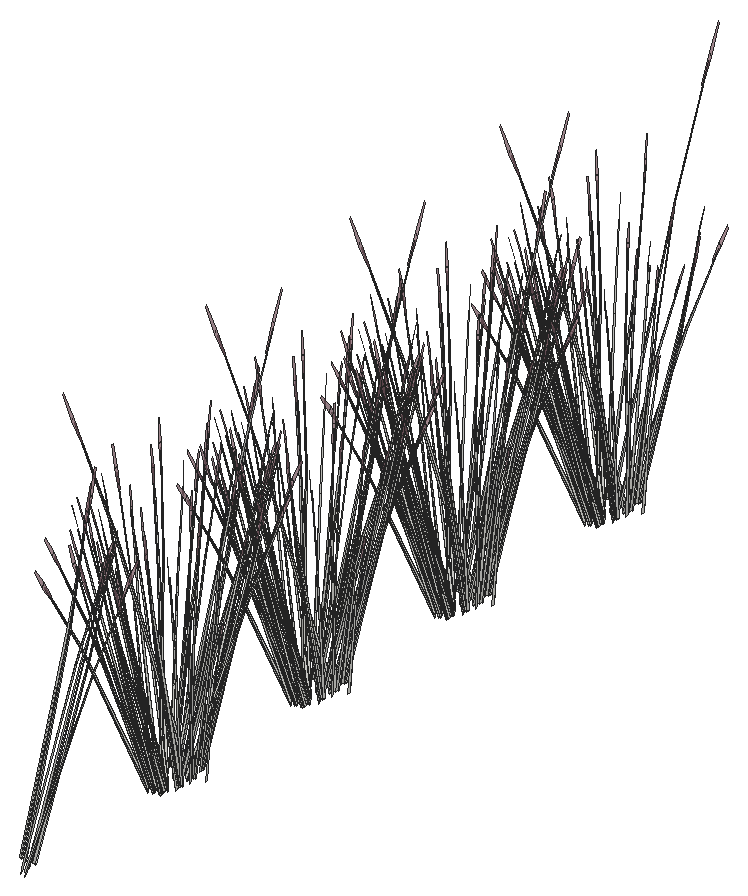
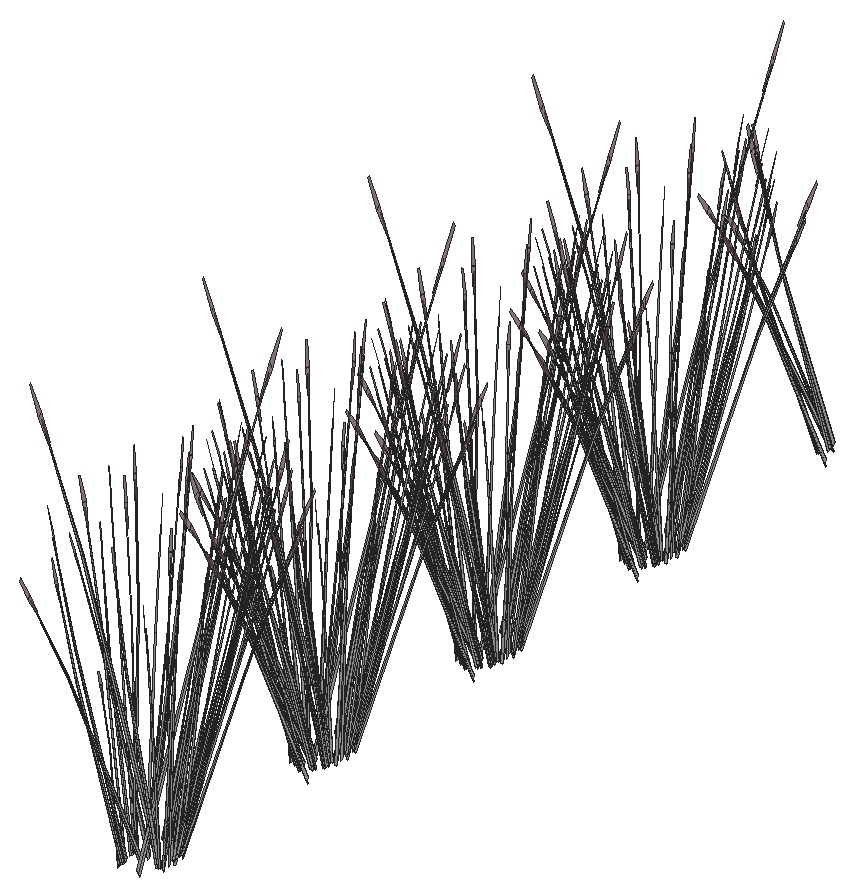
# SketchUp Ruby script. Lengths in inches.
U = 1.inch
M = Sketchup.active_model
def pt(a) = Geom::Point3d.new(a.map { |v| v * U })
def face(e, loops, mat)
  f = e.add_face(loops[0].map { |a| pt(a) })
  loops[1..].each { |l| e.add_face(l.map { |a| pt(a) }).erase! }
  f.material = f.back_material = mat if mat
  f
end
# faces: each face lists its corners as indices into pts; further lists are holes
def faces(e, pts, list, mat = nil) = list.each { |f| face(e, (f[0].is_a?(Array) ? f : [f]).map { |l| l.map { |i| pts[i] } }, mat) }
# xy, xz, yz: faces in a plane at the given z, y or x. An outline is a flat list of corners, or four numbers for a rectangle; further outlines are holes
def ring(l) = l.size == 4 ? [[l[0], l[1]], [l[2], l[1]], [l[2], l[3]], [l[0], l[3]]] : l.each_slice(2).to_a
def flat(e, list, mat, &to3) = list.each { |f| face(e, (f[0].is_a?(Array) ? f : [f]).map { |l| ring(l).map { |u, v| to3.(u, v) } }, mat) }
def xy(e, z, list, mat = nil) = flat(e, list, mat) { |x, y| [x, y, z] }
def xz(e, y, list, mat = nil) = flat(e, list, mat) { |x, z| [x, y, z] }
def yz(e, x, list, mat = nil) = flat(e, list, mat) { |y, z| [x, y, z] }
def lines(e, pts, list) = list.each { |a, b| e.add_line(pt(pts[a]), pt(pts[b])) }
# prism: a flat outline (further loops are holes) pulled along v
def prism(e, loops, v, mat = nil)
  f = face(e, loops, mat); d = Geom::Vector3d.new(v.map { |x| x * U })
  f.pushpull(f.normal.samedirection?(d) ? d.length : -d.length)
end
def box(e, o, s, mat = nil) = prism(e, [[o, [o[0] + s[0], o[1], o[2]], [o[0] + s[0], o[1] + s[1], o[2]], [o[0], o[1] + s[1], o[2]]]], [0, 0, s[2]], mat)
def at(x, y, z, deg = 0) = Geom::Transformation.translation(pt([x, y, z])) * Geom::Transformation.rotation(ORIGIN, Z_AXIS, deg.degrees)
def axes(o, x, y, z) = Geom::Transformation.new([*x, 0, *y, 0, *z, 0, *pt(o).to_a, 1])
def part(name) = M.definitions.add(name)
# library, detail: a bought-in or finely detailed component or shape, given as its bounding box
def library(name, o, s) = part(name).tap { |d| box(d.entities, o, s) }
def detail(e, o, s) = box(e.add_group.entities, o, s)
def put(e, d, t, mat = nil) = e.add_instance(d, t).tap { |i| i.material = mat if mat }
def group(e, t, mat = nil) = e.add_group.tap { |g| g.transformation = t; g.material = mat if mat }.entities
root = M.entities
M.materials.add("LightPink_Translucent").color = [144, 107, 117]
M.materials["LightPink_Translucent"].alpha = 0.75
c1 = part("blade")
p = [[2.15,0.21,22],[0,0.17,0],[0.09,0.45,0],[2.18,0.31,22],[2.29,0.31,22],[0.38,0.45,0],
  [2.48,0.24,33],[2.49,0.24,33],[2.48,0.22,33]]
faces(c1.entities,p,[[0,1,2,3],[4,5,2,3],[6,3,4,7],[8,0,3,6]])
c2 = part("seeds")
p = [[0.3,-0.1,1.38],[-0.01,-0.03,1.59],[-0.01,-0.03,0.03],[0.14,-0.07,-0.07],[0.29,-0.03,3],[0.15,0.01,3.11]]
faces(c2.entities,p,[[0,1,2,3],[1,0,4,5]],"LightPink_Translucent")
c3 = part("blade with seeds")
put(c3.entities,c1,at(0,0,0))
put(c3.entities,c2,axes([2.4,0.25,30.99],[1.5799,-0.05474,1.17369],[-0.12525,1.92788,0.29478],[-0.07173,-0.02425,1.56792]))
put(root,c3,axes([251.06,64.61,2.83],[0.18323,0.41084,-0.41166],[-0.19356,0.3598,-0.31887],[-0.02788,0.20874,0.78768]))
put(root,c3,axes([251.6,65,2.59],[0.25161,0.15328,-0.37087],[-0.08624,0.52553,-0.28727],[0.02307,0.21159,0.70962]))
put(root,c3,axes([251.74,63.92,2.01],[-0.05851,-0.19632,1.24382],[0.27036,-0.16528,0.10057],[0.0611,0.3082,0.53172]))
put(root,c3,axes([251.48,65.33,2.48],[-0.07716,0.47021,-0.25703],[-0.22512,-0.13715,0.33183],[0.02064,0.18932,0.63492]))
put(root,c3,axes([251,64.42,3.07],[-0.00666,0.56559,-0.57235],[-0.28045,-0.03799,0.06907],[-0.0296,0.23961,0.80965]))
put(root,c3,axes([251.26,64.02,2.01],[-0.00626,-0.23468,1.24382],[0.27152,0.15569,0.10057],[-0.01679,0.33444,0.53172]))
put(root,c3,axes([250.9,65.21,1.63],[0.00562,-0.31565,1.12021],[0.25293,0.16673,0.1548],[-0.02192,0.33641,0.52896]))
put(root,c3,axes([251.1,79.1,2.01],[0.05851,0.19632,1.24382],[-0.27036,0.16528,0.10057],[-0.0611,-0.3082,0.53172]))
put(root,c3,axes([251.84,78.82,2.48],[0.07716,-0.47021,-0.25703],[0.22512,0.13715,0.33183],[-0.02064,-0.18932,0.63492]))
put(root,c3,axes([252.01,79.45,2.01],[-0.04766,0.21017,1.24382],[-0.19993,-0.43493,0.10057],[0.09019,-0.27107,0.53172]))
put(root,c3,axes([251.73,79.15,2.59],[-0.25161,-0.15328,-0.37087],[0.08624,-0.52553,-0.28727],[-0.02307,-0.21159,0.70962]))
put(root,c3,axes([252.27,79.54,2.59],[-0.18323,-0.41084,-0.37087],[0.19356,-0.3598,-0.28727],[0.02788,-0.20874,0.70962]))
put(root,c3,axes([251.94,79.12,2.85],[-0.25047,0.28468,-0.08826],[-0.12309,-0.50526,-0.48986],[-0.03305,-0.21292,0.74434]))
put(root,c3,axes([252.46,79.76,2.85],[-0.2813,-0.0303,-0.08826],[0.00769,-0.57361,-0.48986],[0.01954,-0.22092,0.74434]))
put(root,c3,axes([252.44,79.39,2.48],[0.17318,-0.32193,-0.25703],[0.16394,0.36759,0.33183],[0.02494,-0.18677,0.63492]))
put(root,c3,axes([251.19,79,2.48],[-0.03953,-0.49251,-0.25703],[0.22598,-0.13005,0.33183],[-0.0607,-0.14114,0.63492]))
put(root,c3,axes([250.71,79.71,2.01],[0.09507,0.10535,1.24382],[-0.19675,0.44195,0.10057],[-0.12263,-0.19937,0.53172]))
put(root,c3,axes([251.17,79.4,2.59],[-0.25257,0.14535,-0.37087],[-0.04418,-0.55045,-0.28727],[-0.06784,-0.15774,0.70962]))
put(root,c3,axes([252.65,80.49,2.59],[-0.06575,-0.55831,-0.37087],[0.24901,-0.09767,-0.28727],[0.07136,-0.14996,0.70962]))
put(root,c3,axes([252.77,80.89,2.85],[-0.23676,-0.33715,-0.08826],[0.1364,-0.48826,-0.48986],[0.06689,-0.16972,0.74434]))
put(root,c3,axes([251.79,82.73,1.61],[0.22119,0.24656,1.09782],[-0.21669,0.53118,0.43413],[-0.09706,-0.31482,0.92034]))
put(root,c3,axes([252.84,80.55,2.48],[0.2228,-0.08739,-0.25703],[0.05883,0.49954,0.33183],[0.06385,-0.13418,0.63492]))
put(root,c3,axes([250.67,79.86,2.48],[-0.14563,-0.38283,-0.25703],[0.16629,-0.3624,0.33183],[-0.08449,-0.05514,0.63492]))
put(root,c3,axes([250.74,80.24,2.59],[-0.18586,0.40503,-0.37087],[-0.16277,-0.42787,-0.28727],[-0.09443,-0.06163,0.70962]))
put(root,c3,axes([250.84,79.82,2.85],[-0.0137,0.62183,-0.08826],[-0.25949,-0.017,-0.48986],[-0.09994,-0.0432,0.74434]))
put(root,c3,axes([252.78,82.21,2.85],[-0.12878,-0.55367,-0.08826],[0.22857,-0.27208,-0.48986],[0.09632,-0.07305,0.74434]))
put(root,c3,axes([252.77,81.73,2.59],[0.06934,-0.55619,-0.37087],[0.23774,0.19064,-0.28727],[0.09572,-0.051,0.70962]))
put(root,c3,axes([250.51,80.68,2.01],[0.10617,-0.01385,1.24382],[-0.07043,0.60021,0.10057],[-0.1513,-0.03712,0.53172]))
put(root,c3,axes([252.91,81.98,2.48],[0.21272,0.17057,-0.25703],[-0.06204,0.49764,0.33183],[0.08564,-0.04563,0.63492]))
put(root,c3,axes([250.41,81.19,2.48],[-0.21272,-0.17057,-0.25703],[0.06204,-0.49764,0.33183],[-0.08564,0.04563,0.63492]))
put(root,c3,axes([252.33,81.37,2.01],[-0.10617,0.01385,1.24382],[0.07043,-0.60021,0.10057],[0.1513,0.03712,0.53172]))
put(root,c3,axes([251.0625,81.11,1.62],[0.07276,-0.08845,1.2851],[0.02509,0.61759,0.10057],[-0.15759,0.08195,0.4593]))
put(root,c3,axes([250.56,81.44,2.59],[-0.06934,0.55619,-0.37087],[-0.23774,-0.19064,-0.28727],[-0.09572,0.051,0.70962]))
put(root,c3,axes([250.55,80.97,2.85],[0.12878,0.55367,-0.08826],[-0.22857,0.27208,-0.48986],[-0.09632,0.07305,0.74434]))
put(root,c3,axes([253.09,83.37,2.04],[-0.04899,-0.514,-0.02534],[0.23154,-0.11817,-0.1149],[0.04835,0.03259,0.37899]))
put(root,c3,axes([252.49,83.36,2.85],[0.0137,-0.62183,-0.08826],[0.25949,0.017,-0.48986],[0.09994,0.0432,0.74434]))
put(root,c3,axes([250.55,81.73,2.01],[0.08881,-0.12933,1.24382],[0.07477,0.59764,0.10057],[-0.13942,0.13507,0.53172]))
put(root,c3,axes([252.66,83.3125,2.48],[0.14563,0.38283,-0.25703],[-0.16629,0.3624,0.33183],[0.08449,0.05514,0.63492]))
put(root,c3,axes([250.49,82.625,2.48],[-0.2228,0.08739,-0.25703],[-0.05883,-0.49954,0.33183],[-0.06385,0.13418,0.63492]))
put(root,c3,axes([252.13,82.33,2.01],[-0.09507,-0.10535,1.24382],[0.19675,-0.44195,0.10057],[0.12263,0.19937,0.53172]))
put(root,c3,axes([252.15,80.94,2.44],[-0.22117,-0.3177,1.00363],[0.23354,-0.49464,0.43304],[0.07136,0.29809,0.97011]))
put(root,c3,axes([250.56,82.28,2.85],[0.23676,0.33715,-0.08826],[-0.1364,0.48826,-0.48986],[-0.06689,0.16972,0.74434]))
put(root,c3,axes([251.98,84.03,2.85],[0.15252,-0.52338,-0.08826],[0.22088,0.30152,-0.48986],[0.07678,0.14787,0.74434]))
put(root,c3,axes([250.875,82.13,2.01],[0.06393,-0.18788,1.24382],[0.16142,0.50711,0.10057],[-0.11071,0.23094,0.53172]))
put(root,c3,axes([250.67,82.68,2.59],[0.06575,0.55831,-0.37087],[-0.24901,0.09767,-0.28727],[-0.07136,0.14996,0.70962]))
put(root,c3,axes([252.16,83.77,2.59],[0.25257,-0.14535,-0.37087],[0.04418,0.55045,-0.28727],[0.06784,0.15774,0.70962]))
put(root,c3,axes([250.83,82.6,2.01],[0.04766,-0.21017,1.24382],[0.19993,0.43493,0.10057],[-0.09019,0.27107,0.53172]))
put(root,c3,axes([250.88,83.78,2.48],[-0.17318,0.32193,-0.25703],[-0.16394,-0.36759,0.33183],[-0.02494,0.18677,0.63492]))
put(root,c3,axes([251.38,84.05,2.85],[0.25047,-0.28468,-0.08826],[0.12309,0.50526,-0.48986],[0.03305,0.21292,0.74434]))
put(root,c3,axes([251.06,83.63,2.83],[0.18323,0.41084,-0.41166],[-0.19356,0.3598,-0.31887],[-0.02788,0.20874,0.78768]))
put(root,c3,axes([251.6,84.03,2.59],[0.25161,0.15328,-0.37087],[-0.08624,0.52553,-0.28727],[0.02307,0.21159,0.70962]))
put(root,c3,axes([251.74,82.94,2.01],[-0.05851,-0.19632,1.24382],[0.27036,-0.16528,0.10057],[0.0611,0.3082,0.53172]))
put(root,c3,axes([251.48,84.35,2.48],[-0.07716,0.47021,-0.25703],[-0.22512,-0.13715,0.33183],[0.02064,0.18932,0.63492]))
put(root,c3,axes([251,83.44,3.07],[-0.00666,0.56559,-0.57235],[-0.28045,-0.03799,0.06907],[-0.0296,0.23961,0.80965]))
put(root,c3,axes([251.26,83.04,2.01],[-0.00626,-0.23468,1.24382],[0.27152,0.15569,0.10057],[-0.01679,0.33444,0.53172]))
put(root,c3,axes([250.9,84.24,1.63],[0.00562,-0.31565,1.12021],[0.25293,0.16673,0.1548],[-0.02192,0.33641,0.52896]))
put(root,c3,axes([251.1,95.68,2.01],[0.05851,0.19632,1.24382],[-0.27036,0.16528,0.10057],[-0.0611,-0.3082,0.53172]))
put(root,c3,axes([251.82,95.82,2.81],[-0.12216,-0.49718,-0.51563],[0.25147,-0.27708,0.06223],[-0.02857,-0.24022,0.72942]))
put(root,c3,axes([252.33,96.31,2.81],[0.00666,-0.56559,-0.51563],[0.28045,0.03799,0.06223],[0.0296,-0.23961,0.72942]))
put(root,c3,axes([251.84,95.4,2.48],[0.07716,-0.47021,-0.25703],[0.22512,0.13715,0.33183],[-0.02064,-0.18932,0.63492]))
put(root,c3,axes([252.01,96.02,2.01],[-0.04766,0.21017,1.24382],[-0.19993,-0.43493,0.10057],[0.09019,-0.27107,0.53172]))
put(root,c3,axes([251.73,95.72,2.59],[-0.25161,-0.15328,-0.37087],[0.08624,-0.52553,-0.28727],[-0.02307,-0.21159,0.70962]))
put(root,c3,axes([252.27,96.12,2.59],[-0.18323,-0.41084,-0.37087],[0.19356,-0.3598,-0.28727],[0.02788,-0.20874,0.70962]))
put(root,c3,axes([251.94,95.7,2.85],[-0.25047,0.28468,-0.08826],[-0.12309,-0.50526,-0.48986],[-0.03305,-0.21292,0.74434]))
put(root,c3,axes([252.46,96.34,2.85],[-0.2813,-0.0303,-0.08826],[0.00769,-0.57361,-0.48986],[0.01954,-0.22092,0.74434]))
put(root,c3,axes([252.44,95.97,2.48],[0.17318,-0.32193,-0.25703],[0.16394,0.36759,0.33183],[0.02494,-0.18677,0.63492]))
put(root,c3,axes([251.19,95.57,2.48],[-0.03953,-0.49251,-0.25703],[0.22598,-0.13005,0.33183],[-0.0607,-0.14114,0.63492]))
put(root,c3,axes([250.71,96.29,2.01],[0.09507,0.10535,1.24382],[-0.19675,0.44195,0.10057],[-0.12263,-0.19937,0.53172]))
put(root,c3,axes([251.17,95.98,2.59],[-0.25257,0.14535,-0.37087],[-0.04418,-0.55045,-0.28727],[-0.06784,-0.15774,0.70962]))
put(root,c3,axes([252.65,97.07,2.59],[-0.06575,-0.55831,-0.37087],[0.24901,-0.09767,-0.28727],[0.07136,-0.14996,0.70962]))
put(root,c3,axes([252.77,97.47,2.85],[-0.23676,-0.33715,-0.08826],[0.1364,-0.48826,-0.48986],[0.06689,-0.16972,0.74434]))
put(root,c3,axes([251.79,99.31,1.61],[0.22119,0.24656,1.09782],[-0.21669,0.53118,0.43413],[-0.09706,-0.31482,0.92034]))
put(root,c3,axes([252.84,97.125,2.48],[0.2228,-0.08739,-0.25703],[0.05883,0.49954,0.33183],[0.06385,-0.13418,0.63492]))
put(root,c3,axes([250.67,96.4375,2.48],[-0.14563,-0.38283,-0.25703],[0.16629,-0.3624,0.33183],[-0.08449,-0.05514,0.63492]))
put(root,c3,axes([250.74,96.82,2.59],[-0.18586,0.40503,-0.37087],[-0.16277,-0.42787,-0.28727],[-0.09443,-0.06163,0.70962]))
put(root,c3,axes([250.84,96.4,2.85],[-0.0137,0.62183,-0.08826],[-0.25949,-0.017,-0.48986],[-0.09994,-0.0432,0.74434]))
put(root,c3,axes([252.78,98.78,2.85],[-0.12878,-0.55367,-0.08826],[0.22857,-0.27208,-0.48986],[0.09632,-0.07305,0.74434]))
put(root,c3,axes([252.77,98.31,2.59],[0.06934,-0.55619,-0.37087],[0.23774,0.19064,-0.28727],[0.09572,-0.051,0.70962]))
put(root,c3,axes([250.51,97.25,2.01],[0.10617,-0.01385,1.24382],[-0.07043,0.60021,0.10057],[-0.1513,-0.03712,0.53172]))
put(root,c3,axes([252.91,98.5625,2.48],[0.21272,0.17057,-0.25703],[-0.06204,0.49764,0.33183],[0.08564,-0.04563,0.63492]))
put(root,c3,axes([250.41,97.77,2.48],[-0.21272,-0.17057,-0.25703],[0.06204,-0.49764,0.33183],[-0.08564,0.04563,0.63492]))
put(root,c3,axes([252.33,97.94,2.01],[-0.10617,0.01385,1.24382],[0.07043,-0.60021,0.10057],[0.1513,0.03712,0.53172]))
put(root,c3,axes([251.0625,97.69,1.62],[0.07276,-0.08845,1.2851],[0.02509,0.61759,0.10057],[-0.15759,0.08195,0.4593]))
put(root,c3,axes([250.56,98.02,2.59],[-0.06934,0.55619,-0.37087],[-0.23774,-0.19064,-0.28727],[-0.09572,0.051,0.70962]))
put(root,c3,axes([250.55,97.55,2.85],[0.12878,0.55367,-0.08826],[-0.22857,0.27208,-0.48986],[-0.09632,0.07305,0.74434]))
put(root,c3,axes([253.09,99.95,2.04],[-0.04899,-0.514,-0.02534],[0.23154,-0.11817,-0.1149],[0.04835,0.03259,0.37899]))
put(root,c3,axes([252.49,99.93,2.85],[0.0137,-0.62183,-0.08826],[0.25949,0.017,-0.48986],[0.09994,0.0432,0.74434]))
put(root,c3,axes([250.55,98.31,2.01],[0.08881,-0.12933,1.24382],[0.07477,0.59764,0.10057],[-0.13942,0.13507,0.53172]))
put(root,c3,axes([252.5,99.63,2.81],[0.25586,0.01472,-0.51563],[-0.01718,0.61995,0.06223],[0.1084,0.06542,0.72942]))
put(root,c3,axes([252.66,99.89,2.48],[0.14563,0.38283,-0.25703],[-0.16629,0.3624,0.33183],[0.08449,0.05514,0.63492]))
put(root,c3,axes([250.49,99.2,2.48],[-0.2228,0.08739,-0.25703],[-0.05883,-0.49954,0.33183],[-0.06385,0.13418,0.63492]))
put(root,c3,axes([252.13,98.91,2.01],[-0.09507,-0.10535,1.24382],[0.19675,-0.44195,0.10057],[0.12263,0.19937,0.53172]))
put(root,c3,axes([252.15,97.52,2.44],[-0.22117,-0.3177,1.00363],[0.23354,-0.49464,0.43304],[0.07136,0.29809,0.97011]))
put(root,c3,axes([250.56,98.86,2.85],[0.23676,0.33715,-0.08826],[-0.1364,0.48826,-0.48986],[-0.06689,0.16972,0.74434]))
put(root,c3,axes([251.98,100.61,2.85],[0.15252,-0.52338,-0.08826],[0.22088,0.30152,-0.48986],[0.07678,0.14787,0.74434]))
put(root,c3,axes([250.875,98.71,2.01],[0.06393,-0.18788,1.24382],[0.16142,0.50711,0.10057],[-0.11071,0.23094,0.53172]))
put(root,c3,axes([250.67,99.26,2.59],[0.06575,0.55831,-0.37087],[-0.24901,0.09767,-0.28727],[-0.07136,0.14996,0.70962]))
put(root,c3,axes([252.16,100.35,2.59],[0.25257,-0.14535,-0.37087],[0.04418,0.55045,-0.28727],[0.06784,0.15774,0.70962]))
put(root,c3,axes([250.83,99.17,2.01],[0.04766,-0.21017,1.24382],[0.19993,0.43493,0.10057],[-0.09019,0.27107,0.53172]))
put(root,c3,axes([250.88,100.36,2.48],[-0.17318,0.32193,-0.25703],[-0.16394,-0.36759,0.33183],[-0.02494,0.18677,0.63492]))
put(root,c3,axes([251.38,100.63,2.85],[0.25047,-0.28468,-0.08826],[0.12309,0.50526,-0.48986],[0.03305,0.21292,0.74434]))
put(root,c3,axes([251.06,100.21,2.83],[0.18323,0.41084,-0.41166],[-0.19356,0.3598,-0.31887],[-0.02788,0.20874,0.78768]))
put(root,c3,axes([251.6,100.61,2.59],[0.25161,0.15328,-0.37087],[-0.08624,0.52553,-0.28727],[0.02307,0.21159,0.70962]))
put(root,c3,axes([251.74,99.52,2.01],[-0.05851,-0.19632,1.24382],[0.27036,-0.16528,0.10057],[0.0611,0.3082,0.53172]))
put(root,c3,axes([251.48,100.93,2.48],[-0.07716,0.47021,-0.25703],[-0.22512,-0.13715,0.33183],[0.02064,0.18932,0.63492]))
put(root,c3,axes([251,100.02,3.07],[-0.00666,0.56559,-0.57235],[-0.28045,-0.03799,0.06907],[-0.0296,0.23961,0.80965]))
put(root,c3,axes([251.26,99.62,2.01],[-0.00626,-0.23468,1.24382],[0.27152,0.15569,0.10057],[-0.01679,0.33444,0.53172]))
put(root,c3,axes([250.9,100.82,1.63],[0.00562,-0.31565,1.12021],[0.25293,0.16673,0.1548],[-0.02192,0.33641,0.52896]))
put(root,c3,axes([251.1,112.43,2.01],[0.05851,0.19632,1.24382],[-0.27036,0.16528,0.10057],[-0.0611,-0.3082,0.53172]))
put(root,c3,axes([251.82,112.58,2.81],[-0.12216,-0.49718,-0.51563],[0.25147,-0.27708,0.06223],[-0.02857,-0.24022,0.72942]))
put(root,c3,axes([252.33,113.06,2.81],[0.00666,-0.56559,-0.51563],[0.28045,0.03799,0.06223],[0.0296,-0.23961,0.72942]))
put(root,c3,axes([251.84,112.16,2.48],[0.07716,-0.47021,-0.25703],[0.22512,0.13715,0.33183],[-0.02064,-0.18932,0.63492]))
put(root,c3,axes([252.01,112.78,2.01],[-0.04766,0.21017,1.24382],[-0.19993,-0.43493,0.10057],[0.09019,-0.27107,0.53172]))
put(root,c3,axes([251.73,112.48,2.59],[-0.25161,-0.15328,-0.37087],[0.08624,-0.52553,-0.28727],[-0.02307,-0.21159,0.70962]))
put(root,c3,axes([252.27,112.875,2.59],[-0.18323,-0.41084,-0.37087],[0.19356,-0.3598,-0.28727],[0.02788,-0.20874,0.70962]))
put(root,c3,axes([251.94,112.45,2.85],[-0.25047,0.28468,-0.08826],[-0.12309,-0.50526,-0.48986],[-0.03305,-0.21292,0.74434]))
put(root,c3,axes([252.46,113.09,2.85],[-0.2813,-0.0303,-0.08826],[0.00769,-0.57361,-0.48986],[0.01954,-0.22092,0.74434]))
put(root,c3,axes([252.44,112.72,2.48],[0.17318,-0.32193,-0.25703],[0.16394,0.36759,0.33183],[0.02494,-0.18677,0.63492]))
put(root,c3,axes([251.27,112.72,2.81],[-0.21825,-0.29555,-0.51563],[0.15511,-0.5179,0.06223],[-0.07907,-0.17646,0.72942]))
put(root,c3,axes([251.19,112.33,2.48],[-0.03953,-0.49251,-0.25703],[0.22598,-0.13005,0.33183],[-0.0607,-0.14114,0.63492]))
put(root,c3,axes([250.71,113.04,2.01],[0.09507,0.10535,1.24382],[-0.19675,0.44195,0.10057],[-0.12263,-0.19937,0.53172]))
put(root,c3,axes([251.17,112.73,2.59],[-0.25257,0.14535,-0.37087],[-0.04418,-0.55045,-0.28727],[-0.06784,-0.15774,0.70962]))
put(root,c3,axes([252.66,114.05,2.81],[0.1337,-0.48245,-0.51563],[0.23429,0.34287,0.06223],[0.07983,-0.1748,0.72942]))
put(root,c3,axes([252.65,113.82,2.59],[-0.06575,-0.55831,-0.37087],[0.24901,-0.09767,-0.28727],[0.07136,-0.14996,0.70962]))
put(root,c3,axes([252.77,114.22,2.85],[-0.23676,-0.33715,-0.08826],[0.1364,-0.48826,-0.48986],[0.06689,-0.16972,0.74434]))
put(root,c3,axes([251.79,116.0625,1.61],[0.22119,0.24656,1.09782],[-0.21669,0.53118,0.43413],[-0.09706,-0.31482,0.92034]))
put(root,c3,axes([252.84,113.88,2.48],[0.2228,-0.08739,-0.25703],[0.05883,0.49954,0.33183],[0.06385,-0.13418,0.63492]))
put(root,c3,axes([250.67,113.19,2.48],[-0.14563,-0.38283,-0.25703],[0.16629,-0.3624,0.33183],[-0.08449,-0.05514,0.63492]))
put(root,c3,axes([250.82,113.45,2.81],[-0.25586,-0.01472,-0.51563],[0.01718,-0.61995,0.06223],[-0.1084,-0.06542,0.72942]))
put(root,c3,axes([250.74,113.58,2.59],[-0.18586,0.40503,-0.37087],[-0.16277,-0.42787,-0.28727],[-0.09443,-0.06163,0.70962]))
put(root,c3,axes([250.84,113.15,2.85],[-0.0137,0.62183,-0.08826],[-0.25949,-0.017,-0.48986],[-0.09994,-0.0432,0.74434]))
put(root,c3,axes([252.78,115.54,2.85],[-0.12878,-0.55367,-0.08826],[0.22857,-0.27208,-0.48986],[0.09632,-0.07305,0.74434]))
put(root,c3,axes([252.77,115.0625,2.59],[0.06934,-0.55619,-0.37087],[0.23774,0.19064,-0.28727],[0.09572,-0.051,0.70962]))
put(root,c3,axes([250.51,114.01,2.01],[0.10617,-0.01385,1.24382],[-0.07043,0.60021,0.10057],[-0.1513,-0.03712,0.53172]))
put(root,c3,axes([252.72,115.26,2.81],[0.22491,-0.27005,-0.51563],[0.12534,0.55588,0.06223],[0.10867,-0.06315,0.72942]))
put(root,c3,axes([252.91,115.32,2.48],[0.21272,0.17057,-0.25703],[-0.06204,0.49764,0.33183],[0.08564,-0.04563,0.63492]))
put(root,c3,axes([250.41,114.52,2.48],[-0.21272,-0.17057,-0.25703],[0.06204,-0.49764,0.33183],[-0.08564,0.04563,0.63492]))
put(root,c3,axes([252.33,114.7,2.01],[-0.10617,0.01385,1.24382],[0.07043,-0.60021,0.10057],[0.1513,0.03712,0.53172]))
put(root,c3,axes([251.0625,114.44,1.62],[0.07276,-0.08845,1.2851],[0.02509,0.61759,0.10057],[-0.15759,0.08195,0.4593]))
put(root,c3,axes([250.56,114.78,2.59],[-0.06934,0.55619,-0.37087],[-0.23774,-0.19064,-0.28727],[-0.09572,0.051,0.70962]))
put(root,c3,axes([250.55,114.3,2.85],[0.12878,0.55367,-0.08826],[-0.22857,0.27208,-0.48986],[-0.09632,0.07305,0.74434]))
put(root,c3,axes([253.09,116.7,2.04],[-0.04899,-0.514,-0.02534],[0.23154,-0.11817,-0.1149],[0.04835,0.03259,0.37899]))
put(root,c3,axes([252.49,116.6875,2.85],[0.0137,-0.62183,-0.08826],[0.25949,0.017,-0.48986],[0.09994,0.0432,0.74434]))
put(root,c3,axes([250.55,115.0625,2.01],[0.08881,-0.12933,1.24382],[0.07477,0.59764,0.10057],[-0.13942,0.13507,0.53172]))
put(root,c3,axes([252.5,116.39,2.81],[0.25586,0.01472,-0.51563],[-0.01718,0.61995,0.06223],[0.1084,0.06542,0.72942]))
put(root,c3,axes([252.66,116.64,2.48],[0.14563,0.38283,-0.25703],[-0.16629,0.3624,0.33183],[0.08449,0.05514,0.63492]))
put(root,c3,axes([250.49,115.96,2.48],[-0.2228,0.08739,-0.25703],[-0.05883,-0.49954,0.33183],[-0.06385,0.13418,0.63492]))
put(root,c3,axes([252.13,115.66,2.01],[-0.09507,-0.10535,1.24382],[0.19675,-0.44195,0.10057],[0.12263,0.19937,0.53172]))
put(root,c3,axes([252.15,114.28,2.44],[-0.22117,-0.3177,1.00363],[0.23354,-0.49464,0.43304],[0.07136,0.29809,0.97011]))
put(root,c3,axes([250.56,115.62,2.85],[0.23676,0.33715,-0.08826],[-0.1364,0.48826,-0.48986],[-0.06689,0.16972,0.74434]))
put(root,c3,axes([251.98,117.36,2.85],[0.15252,-0.52338,-0.08826],[0.22088,0.30152,-0.48986],[0.07678,0.14787,0.74434]))
put(root,c3,axes([250.875,115.47,2.01],[0.06393,-0.18788,1.24382],[0.16142,0.50711,0.10057],[-0.11071,0.23094,0.53172]))
put(root,c3,axes([250.67,116.02,2.59],[0.06575,0.55831,-0.37087],[-0.24901,0.09767,-0.28727],[-0.07136,0.14996,0.70962]))
put(root,c3,axes([252.16,117.1,2.59],[0.25257,-0.14535,-0.37087],[0.04418,0.55045,-0.28727],[0.06784,0.15774,0.70962]))
put(root,c3,axes([250.83,115.93,2.01],[0.04766,-0.21017,1.24382],[0.19993,0.43493,0.10057],[-0.09019,0.27107,0.53172]))
put(root,c3,axes([250.88,117.11,2.48],[-0.17318,0.32193,-0.25703],[-0.16394,-0.36759,0.33183],[-0.02494,0.18677,0.63492]))
put(root,c3,axes([251.38,117.39,2.85],[0.25047,-0.28468,-0.08826],[0.12309,0.50526,-0.48986],[0.03305,0.21292,0.74434]))
put(root,c3,axes([251.06,116.96,2.83],[0.18323,0.41084,-0.41166],[-0.19356,0.3598,-0.31887],[-0.02788,0.20874,0.78768]))
put(root,c3,axes([251.6,117.36,2.59],[0.25161,0.15328,-0.37087],[-0.08624,0.52553,-0.28727],[0.02307,0.21159,0.70962]))
put(root,c3,axes([251.74,116.28,2.01],[-0.05851,-0.19632,1.24382],[0.27036,-0.16528,0.10057],[0.0611,0.3082,0.53172]))
put(root,c3,axes([251.48,117.68,2.48],[-0.07716,0.47021,-0.25703],[-0.22512,-0.13715,0.33183],[0.02064,0.18932,0.63492]))
put(root,c3,axes([251,116.77,3.07],[-0.00666,0.56559,-0.57235],[-0.28045,-0.03799,0.06907],[-0.0296,0.23961,0.80965]))
put(root,c3,axes([251.26,116.375,2.01],[-0.00626,-0.23468,1.24382],[0.27152,0.15569,0.10057],[-0.01679,0.33444,0.53172]))
put(root,c3,axes([251.51,117.26,2.81],[0.12216,0.49718,-0.51563],[-0.25147,0.27708,0.06223],[0.02857,0.24022,0.72942]))
put(root,c3,axes([250.9,117.57,1.63],[0.00562,-0.31565,1.12021],[0.25293,0.16673,0.1548],[-0.02192,0.33641,0.52896]))
put(root,c3,axes([251.1,129.88,2.01],[0.05851,0.19632,1.24382],[-0.27036,0.16528,0.10057],[-0.0611,-0.3082,0.53172]))
put(root,c3,axes([251.82,130.02,2.81],[-0.12216,-0.49718,-0.51563],[0.25147,-0.27708,0.06223],[-0.02857,-0.24022,0.72942]))
put(root,c3,axes([252.33,130.51,2.81],[0.00666,-0.56559,-0.51563],[0.28045,0.03799,0.06223],[0.0296,-0.23961,0.72942]))
put(root,c3,axes([251.84,129.6,2.48],[0.07716,-0.47021,-0.25703],[0.22512,0.13715,0.33183],[-0.02064,-0.18932,0.63492]))
put(root,c3,axes([252.01,130.22,2.01],[-0.04766,0.21017,1.24382],[-0.19993,-0.43493,0.10057],[0.09019,-0.27107,0.53172]))
put(root,c3,axes([251.73,129.92,2.59],[-0.25161,-0.15328,-0.37087],[0.08624,-0.52553,-0.28727],[-0.02307,-0.21159,0.70962]))
put(root,c3,axes([252.27,130.32,2.59],[-0.18323,-0.41084,-0.37087],[0.19356,-0.3598,-0.28727],[0.02788,-0.20874,0.70962]))
put(root,c3,axes([251.94,129.9,2.85],[-0.25047,0.28468,-0.08826],[-0.12309,-0.50526,-0.48986],[-0.03305,-0.21292,0.74434]))
put(root,c3,axes([252.46,130.54,2.85],[-0.2813,-0.0303,-0.08826],[0.00769,-0.57361,-0.48986],[0.01954,-0.22092,0.74434]))
put(root,c3,axes([252.44,130.17,2.48],[0.17318,-0.32193,-0.25703],[0.16394,0.36759,0.33183],[0.02494,-0.18677,0.63492]))
put(root,c3,axes([251.27,130.16,2.81],[-0.21825,-0.29555,-0.51563],[0.15511,-0.5179,0.06223],[-0.07907,-0.17646,0.72942]))
put(root,c3,axes([251.19,129.77,2.48],[-0.03953,-0.49251,-0.25703],[0.22598,-0.13005,0.33183],[-0.0607,-0.14114,0.63492]))
put(root,c3,axes([250.71,130.49,2.01],[0.09507,0.10535,1.24382],[-0.19675,0.44195,0.10057],[-0.12263,-0.19937,0.53172]))
put(root,c3,axes([251.17,130.18,2.59],[-0.25257,0.14535,-0.37087],[-0.04418,-0.55045,-0.28727],[-0.06784,-0.15774,0.70962]))
put(root,c3,axes([252.66,131.49,2.81],[0.1337,-0.48245,-0.51563],[0.23429,0.34287,0.06223],[0.07983,-0.1748,0.72942]))
put(root,c3,axes([252.65,131.27,2.59],[-0.06575,-0.55831,-0.37087],[0.24901,-0.09767,-0.28727],[0.07136,-0.14996,0.70962]))
put(root,c3,axes([252.77,131.67,2.85],[-0.23676,-0.33715,-0.08826],[0.1364,-0.48826,-0.48986],[0.06689,-0.16972,0.74434]))
put(root,c3,axes([251.79,133.51,1.61],[0.22119,0.24656,1.09782],[-0.21669,0.53118,0.43413],[-0.09706,-0.31482,0.92034]))
put(root,c3,axes([252.84,131.33,2.48],[0.2228,-0.08739,-0.25703],[0.05883,0.49954,0.33183],[0.06385,-0.13418,0.63492]))
put(root,c3,axes([250.67,130.64,2.48],[-0.14563,-0.38283,-0.25703],[0.16629,-0.3624,0.33183],[-0.08449,-0.05514,0.63492]))
put(root,c3,axes([250.82,130.9,2.81],[-0.25586,-0.01472,-0.51563],[0.01718,-0.61995,0.06223],[-0.1084,-0.06542,0.72942]))
put(root,c3,axes([250.74,131.02,2.59],[-0.18586,0.40503,-0.37087],[-0.16277,-0.42787,-0.28727],[-0.09443,-0.06163,0.70962]))
put(root,c3,axes([250.84,130.6,2.85],[-0.0137,0.62183,-0.08826],[-0.25949,-0.017,-0.48986],[-0.09994,-0.0432,0.74434]))
put(root,c3,axes([252.78,132.98,2.85],[-0.12878,-0.55367,-0.08826],[0.22857,-0.27208,-0.48986],[0.09632,-0.07305,0.74434]))
put(root,c3,axes([252.77,132.51,2.59],[0.06934,-0.55619,-0.37087],[0.23774,0.19064,-0.28727],[0.09572,-0.051,0.70962]))
put(root,c3,axes([250.51,131.45,2.01],[0.10617,-0.01385,1.24382],[-0.07043,0.60021,0.10057],[-0.1513,-0.03712,0.53172]))
put(root,c3,axes([252.72,132.71,2.81],[0.22491,-0.27005,-0.51563],[0.12534,0.55588,0.06223],[0.10867,-0.06315,0.72942]))
put(root,c3,axes([252.91,132.76,2.48],[0.21272,0.17057,-0.25703],[-0.06204,0.49764,0.33183],[0.08564,-0.04563,0.63492]))
put(root,c3,axes([250.41,131.97,2.48],[-0.21272,-0.17057,-0.25703],[0.06204,-0.49764,0.33183],[-0.08564,0.04563,0.63492]))
put(root,c3,axes([252.33,132.15,2.01],[-0.10617,0.01385,1.24382],[0.07043,-0.60021,0.10057],[0.1513,0.03712,0.53172]))
put(root,c3,axes([251.0625,131.89,1.62],[0.07276,-0.08845,1.2851],[0.02509,0.61759,0.10057],[-0.15759,0.08195,0.4593]))
put(root,c3,axes([250.56,132.22,2.59],[-0.06934,0.55619,-0.37087],[-0.23774,-0.19064,-0.28727],[-0.09572,0.051,0.70962]))
put(root,c3,axes([250.55,131.75,2.85],[0.12878,0.55367,-0.08826],[-0.22857,0.27208,-0.48986],[-0.09632,0.07305,0.74434]))
put(root,c3,axes([253.09,134.15,2.04],[-0.04899,-0.514,-0.02534],[0.23154,-0.11817,-0.1149],[0.04835,0.03259,0.37899]))
put(root,c3,axes([252.49,134.13,2.85],[0.0137,-0.62183,-0.08826],[0.25949,0.017,-0.48986],[0.09994,0.0432,0.74434]))
put(root,c3,axes([250.55,132.51,2.01],[0.08881,-0.12933,1.24382],[0.07477,0.59764,0.10057],[-0.13942,0.13507,0.53172]))
put(root,c3,axes([252.5,133.83,2.81],[0.25586,0.01472,-0.51563],[-0.01718,0.61995,0.06223],[0.1084,0.06542,0.72942]))
put(root,c3,axes([252.66,134.09,2.48],[0.14563,0.38283,-0.25703],[-0.16629,0.3624,0.33183],[0.08449,0.05514,0.63492]))
put(root,c3,axes([250.49,133.4,2.48],[-0.2228,0.08739,-0.25703],[-0.05883,-0.49954,0.33183],[-0.06385,0.13418,0.63492]))
put(root,c3,axes([252.13,133.11,2.01],[-0.09507,-0.10535,1.24382],[0.19675,-0.44195,0.10057],[0.12263,0.19937,0.53172]))
put(root,c3,axes([252.15,131.72,2.44],[-0.22117,-0.3177,1.00363],[0.23354,-0.49464,0.43304],[0.07136,0.29809,0.97011]))
put(root,c3,axes([250.56,133.0625,2.85],[0.23676,0.33715,-0.08826],[-0.1364,0.48826,-0.48986],[-0.06689,0.16972,0.74434]))
